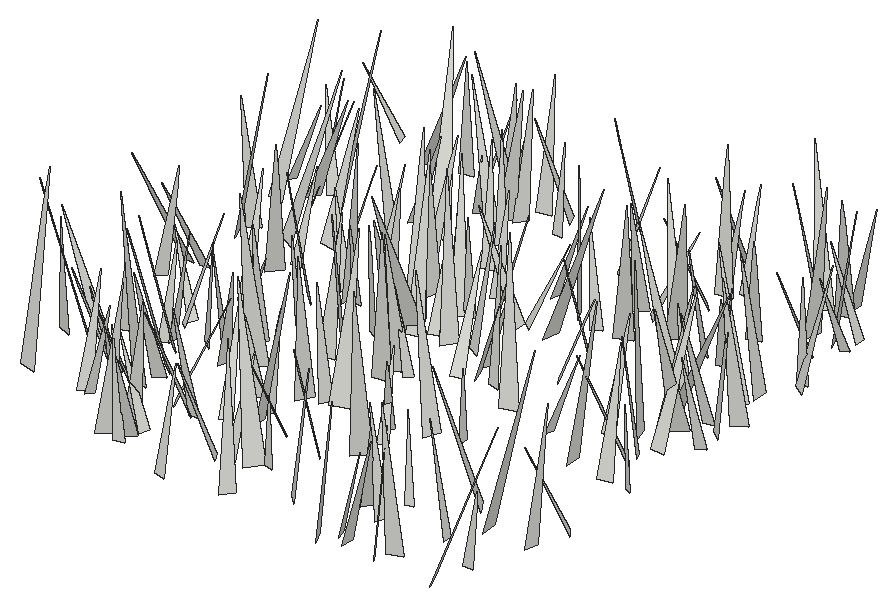
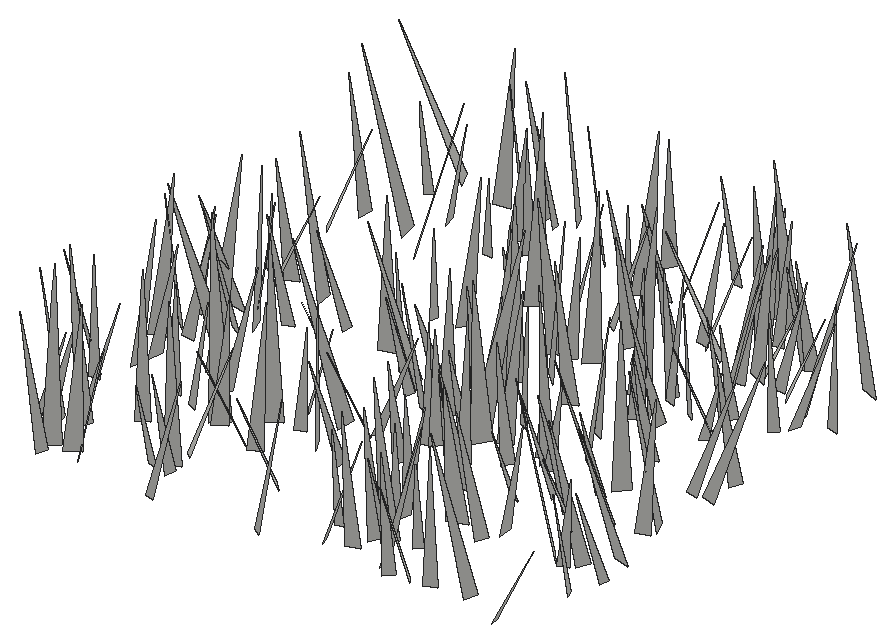
# SketchUp Ruby script. Lengths in inches.
U = 1.inch
M = Sketchup.active_model
def pt(a) = Geom::Point3d.new(a.map { |v| v * U })
def face(e, loops, mat)
  f = e.add_face(loops[0].map { |a| pt(a) })
  loops[1..].each { |l| e.add_face(l.map { |a| pt(a) }).erase! }
  f.material = f.back_material = mat if mat
  f
end
# faces: each face lists its corners as indices into pts; further lists are holes
def faces(e, pts, list, mat = nil) = list.each { |f| face(e, (f[0].is_a?(Array) ? f : [f]).map { |l| l.map { |i| pts[i] } }, mat) }
# xy, xz, yz: faces in a plane at the given z, y or x. An outline is a flat list of corners, or four numbers for a rectangle; further outlines are holes
def ring(l) = l.size == 4 ? [[l[0], l[1]], [l[2], l[1]], [l[2], l[3]], [l[0], l[3]]] : l.each_slice(2).to_a
def flat(e, list, mat, &to3) = list.each { |f| face(e, (f[0].is_a?(Array) ? f : [f]).map { |l| ring(l).map { |u, v| to3.(u, v) } }, mat) }
def xy(e, z, list, mat = nil) = flat(e, list, mat) { |x, y| [x, y, z] }
def xz(e, y, list, mat = nil) = flat(e, list, mat) { |x, z| [x, y, z] }
def yz(e, x, list, mat = nil) = flat(e, list, mat) { |y, z| [x, y, z] }
def lines(e, pts, list) = list.each { |a, b| e.add_line(pt(pts[a]), pt(pts[b])) }
# prism: a flat outline (further loops are holes) pulled along v
def prism(e, loops, v, mat = nil)
  f = face(e, loops, mat); d = Geom::Vector3d.new(v.map { |x| x * U })
  f.pushpull(f.normal.samedirection?(d) ? d.length : -d.length)
end
def box(e, o, s, mat = nil) = prism(e, [[o, [o[0] + s[0], o[1], o[2]], [o[0] + s[0], o[1] + s[1], o[2]], [o[0], o[1] + s[1], o[2]]]], [0, 0, s[2]], mat)
def at(x, y, z, deg = 0) = Geom::Transformation.translation(pt([x, y, z])) * Geom::Transformation.rotation(ORIGIN, Z_AXIS, deg.degrees)
def axes(o, x, y, z) = Geom::Transformation.new([*x, 0, *y, 0, *z, 0, *pt(o).to_a, 1])
def part(name) = M.definitions.add(name)
# library, detail: a bought-in or finely detailed component or shape, given as its bounding box
def library(name, o, s) = part(name).tap { |d| box(d.entities, o, s) }
def detail(e, o, s) = box(e.add_group.entities, o, s)
def put(e, d, t, mat = nil) = e.add_instance(d, t).tap { |i| i.material = mat if mat }
def group(e, t, mat = nil) = e.add_group.tap { |g| g.transformation = t; g.material = mat if mat }.entities
root = M.entities
c1 = part("fur_instance\#9")
p = [[0.8125,0,1.79],[0.67,-0.02,1.48],[0,-0.11,0],[0,0.11,0]]
faces(c1.entities,p,[[0,1,2,3]])
put(root,c1,axes([499.34,279.74,-21.66],[-1.38983,-5.84462,0.0201],[-5.82782,1.38425,-0.46046],[-0.44334,0.12603,5.98992]))
put(root,c1,axes([498.6,291.3,-21.66],[1.7832,7.11152,0.69499],[7.11724,-1.83129,0.47737],[-0.63379,-0.55606,7.31612]))
put(root,c1,axes([497.63,294.57,-21.66],[3.74369,-0.67268,0.40161],[-0.71907,-3.7286,0.45768],[-0.31101,0.52348,3.776]))
put(root,c1,axes([498.79,265.3,-21.66],[-1.48378,-4.80354,1.85374],[-5.06695,1.70492,0.36217],[0.91449,1.65264,5.01442]))
put(root,c1,axes([500.375,304.53,-21.66],[-3.53813,-0.73541,0.01575],[-0.72603,3.50386,0.50526],[0.11809,-0.49152,3.57826]))
put(root,c1,axes([498.56,297.67,-21.66],[3.70099,1.78589,1.07617],[1.91017,-3.78303,-0.29128],[-0.83593,-0.7377,4.09901]))
put(root,c1,axes([501.26,266.79,-21.66],[-5.40823,0.65228,0.52882],[0.69912,5.40686,0.48075],[0.46513,-0.5426,5.42617]))
put(root,c1,axes([500.03,286.84,-21.66],[1.93856,-5.12728,2.24723],[-5.46022,-2.25638,-0.43794],[-1.23493,1.9279,5.46399]))
put(root,c1,axes([499.18,276.6,-21.66],[4.20018,-2.603,1.54886],[-2.85846,-4.28223,0.55487],[-1.0019,1.30501,4.91012]))
put(root,c1,axes([500.125,259.14,-21.66],[2.12447,7.8086,2.15105],[8.03257,-2.31646,0.47574],[-1.03873,-1.94278,8.07844]))
put(root,c1,axes([500.91,279.75,-21.66],[-0.25255,-4.7231,0.0991],[-4.68784,0.23828,-0.59045],[-0.58449,0.12972,4.69284]))
put(root,c1,axes([499.63,285.33,-21.66],[6.18065,2.99725,1.89028],[2.99834,-6.44896,0.42186],[-1.88855,-0.42956,6.85609]))
put(root,c1,axes([502.44,264.21,-21.66],[-5.20648,-5.71637,1.32602],[-5.85189,5.18966,-0.6046],[0.43665,1.3904,7.70836]))
put(root,c1,axes([501.63,294.57,-21.66],[-2.18486,3.79279,1.02862],[3.92891,2.13324,0.47945],[0.08359,-1.13179,4.35074]))
put(root,c1,axes([501.34,292.31,-21.66],[4.04394,2.43918,0.42992],[2.39305,-4.06014,0.52577],[-0.63852,0.23141,4.69325]))
put(root,c1,axes([500.51,293.5,-21.66],[5.28357,-2.5058,0.04843],[-2.504,-5.27298,0.35108],[0.10676,0.33794,5.83712]))
put(root,c1,axes([502.1875,268.22,-21.66],[2.0816,-3.74764,1.04429],[-3.88491,-2.06538,0.3318],[-0.20701,1.076,4.27408]))
put(root,c1,axes([504.64,263.61,-21.66],[-3.58425,-2.16039,0.18109],[-2.16614,3.55434,-0.47063],[-0.08907,0.49634,4.15845]))
put(root,c1,axes([505.53,272.56,-21.66],[-3.05082,2.35934,0.28628],[2.37608,3.01778,0.45074],[-0.05159,-0.53147,3.83025]))
put(root,c1,axes([502.97,293.86,-21.66],[5.7382,5.20942,1.87337],[5.41352,-5.84467,-0.3291],[-1.15821,-1.50876,7.74318]))
put(root,c1,axes([503.29,286.72,-21.66],[3.5873,6.66463,1.07182],[6.75002,-3.55215,-0.50434],[-0.05834,-1.18311,7.55193]))
put(root,c1,axes([505.76,263.01,-21.66],[0.4513,-4.46287,0.47479],[-4.46772,-0.49211,-0.3789],[-0.42669,0.43236,4.4696]))
put(root,c1,axes([507.15,268.3125,-21.66],[2.82941,3.82153,3.56935],[4.50896,-3.83832,0.53527],[-2.64833,-2.45217,4.72474]))
put(root,c1,axes([505.79,258.96,-21.66],[-2.49427,4.27012,1.59064],[4.35584,2.76683,-0.59729],[1.33819,-1.04698,4.90903]))
put(root,c1,axes([505.79,268.68,-21.66],[2.7326,-2.75522,2.01665],[-3.2693,-2.85632,0.52755],[-0.98478,1.83723,3.84448]))
put(root,c1,axes([505.4,271.625,-21.66],[2.99735,3.72962,0.28981],[3.68324,-3.00724,0.60693],[-0.65404,0.15682,4.74613]))
put(root,c1,axes([506.6875,277.54,-21.66],[-1.85743,4.94831,0.92273],[4.99711,1.93095,-0.29602],[0.60509,-0.75691,5.27714]))
put(root,c1,axes([506.23,284.25,-21.66],[-0.0874,4.08723,0.80677],[4.1529,0.14964,-0.30818],[0.33125,-0.79758,4.07653]))
put(root,c1,axes([506.19,269.28,-21.66],[4.45017,0.43948,1.54669],[0.28501,-4.6951,0.51402],[-1.58245,0.39027,4.44218]))
put(root,c1,axes([505.49,282.6,-21.66],[5.14782,-4.26055,1.16689],[-4.27581,-5.25589,-0.32723],[-1.10966,0.4872,6.67423]))
put(root,c1,axes([508.16,261.84,-21.66],[-3.2308,-2.41105,0.08917],[-2.40238,3.20101,-0.49122],[-0.22293,0.4467,4.00124]))
put(root,c1,axes([504.15,302.67,-21.66],[6.51578,-0.90085,0.09034],[-0.89347,-6.50413,-0.41604],[-0.1463,-0.39981,6.56459]))
put(root,c1,axes([506.24,288.07,-21.66],[-0.03084,5.75903,1.17934],[5.85206,0.14189,-0.53988],[0.55736,-1.17118,5.73375]))
put(root,c1,axes([508.36,293.22,-21.66],[-5.56537,0.35389,1.01892],[0.25962,5.63719,-0.53984],[1.04691,0.48332,5.55042]))
put(root,c1,axes([506.39,258.94,-21.66],[3.89931,-1.45547,0.98195],[-1.58431,-3.9476,0.44006],[-0.75669,0.76505,4.13877]))
put(root,c1,axes([508.73,265.49,-21.66],[-4.07714,-4.72232,1.18622],[-4.85623,4.056,-0.54439],[0.3528,1.25658,6.21506]))
put(root,c1,axes([508.3125,262.53,-21.66],[-2.90002,-7.26429,3.03178],[-7.85451,2.88308,-0.60516],[0.51793,3.0479,7.79832]))
put(root,c1,axes([507.6,303.32,-21.66],[1.5026,-5.2869,1.47769],[-5.48951,-1.44343,0.41772],[0.01326,1.53554,5.48039]))
put(root,c1,axes([508.99,264.18,-21.66],[1.67149,-5.33301,0.8085],[-5.34441,-1.75188,-0.5067],[-0.72935,0.6152,5.5658]))
put(root,c1,axes([508.61,270.39,-21.66],[2.85129,3.39796,1.84964],[3.79237,-2.9092,-0.50161],[-0.76499,-1.75715,4.40731]))
put(root,c1,axes([510.35,280.75,-21.66],[-3.95359,-4.39819,1.62013],[-4.4402,4.19331,0.54823],[1.50116,0.81969,5.8885]))
put(root,c1,axes([509.02,286.45,-21.66],[4.30125,1.72732,0.68489],[1.69718,-4.35514,0.32517],[-0.75649,0.05042,4.6237]))
put(root,c1,axes([509.4,303.49,-21.66],[3.16954,2.48643,0.53995],[2.54162,-3.13416,-0.48689],[-0.1185,-0.71733,3.99891]))
put(root,c1,axes([510.1,257.78,-21.66],[0.02895,-4.95019,0.58964],[-4.94989,0.0415,0.59139],[0.59214,0.58889,4.91483]))
put(root,c1,axes([512.21,294.27,-21.66],[-3.14428,7.71271,0.49149],[7.72648,3.12546,0.38342],[-0.17032,-0.59964,8.32018]))
put(root,c1,axes([509.08,295.21,-21.66],[4.36325,-2.68491,0.18726],[-2.69098,-4.34538,0.39756],[0.04948,0.43666,5.1077]))
put(root,c1,axes([511.69,283.57,-21.66],[-3.05036,2.77962,1.08054],[2.93347,3.07501,0.37088],[0.53722,-1.00823,4.11016]))
put(root,c1,axes([511.12,288.67,-21.66],[1.03899,3.82207,0.22987],[3.79032,-1.06041,0.49963],[-0.54276,-0.08876,3.92914]))
put(root,c1,axes([509.55,272.8125,-21.66],[4.16125,-1.09144,0.28201],[-1.11074,-4.15389,0.31328],[-0.19241,0.37504,4.29058]))
put(root,c1,axes([512.47,302.75,-21.66],[-6.25427,-0.78477,1.30734],[-0.71032,6.38344,0.43371],[1.34924,-0.27711,6.28838]))
put(root,c1,axes([511.19,269.66,-21.66],[-1.65824,-4.82946,1.36253],[-4.95542,1.80194,0.35604],[0.78993,1.16588,5.09379]))
put(root,c1,axes([510.92,272.39,-21.66],[4.15437,2.45212,1.76514],[2.75663,-4.30471,-0.50784],[-1.23677,-1.35794,4.79727]))
put(root,c1,axes([512.28,277.05,-21.66],[0.90627,3.33198,1.59944],[3.57947,-1.20149,0.47479],[-0.9207,-1.39138,3.42023]))
put(root,c1,axes([511.11,303.9375,-21.66],[3.01124,-3.84874,1.35887],[-4.04465,-3.04041,0.35153],[-0.54781,1.29229,4.87409]))
put(root,c1,axes([513.33,256.85,-21.66],[-4.0044,1.49429,0.5536],[1.5481,4.00291,0.3933],[0.37782,-0.56428,4.25599]))
put(root,c1,axes([511.1,254.85,-21.66],[5.02607,-4.57327,2.19343],[-4.92834,-5.13329,0.59007],[-1.19892,1.92923,6.76964]))
put(root,c1,axes([511.59,273.23,-21.66],[4.45698,-3.93649,1.376],[-3.92382,-4.64074,-0.56675],[-1.41173,0.47074,5.91941]))
put(root,c1,axes([512.8125,254.48,-21.66],[-0.34045,4.62028,2.07312],[5.05885,0.21591,0.34957],[-0.23002,-2.08976,4.6196]))
put(root,c1,axes([511.52,268.94,-21.66],[4.68677,-2.0034,0.66372],[-1.95488,-4.73014,-0.47351],[-0.79535,-0.17932,5.07496]))
put(root,c1,axes([511.71,257.5,-21.66],[3.13383,-5.16211,1.39491],[-5.34355,-3.08346,0.59403],[-0.19921,1.50298,6.00961]))
put(root,c1,axes([512,299.24,-21.66],[1.97582,-3.11414,0.08334],[-3.10691,-1.9626,0.3224],[0.22782,0.24287,3.67393]))
put(root,c1,axes([514.36,261.22,-21.66],[-3.87512,-3.17972,0.32504],[-3.163,3.88842,0.32938],[0.4601,-0.04943,5.00187]))
put(root,c1,axes([512.65,282.7,-21.66],[7.01983,-0.71592,2.31882],[-0.6287,-7.39114,-0.37866],[-2.34397,-0.1616,7.04608]))
put(root,c1,axes([513,255.68,-21.66],[2.62732,-3.98087,0.28129],[-3.95197,-2.64215,-0.47983],[-0.55532,-0.03119,4.74551]))
put(root,c1,axes([513.67,270.21,-21.66],[3.74176,-6.61768,2.63887],[-6.89022,-4.11933,-0.5604],[-1.81167,1.99888,7.58159]))
put(root,c1,axes([515.92,296.26,-21.66],[-6.2227,2.39174,0.32304],[2.36421,6.22042,-0.51348],[0.48507,0.36431,6.64671]))
put(root,c1,axes([513.51,282.51,-21.66],[0.0585,-4.06465,0.78718],[-4.11626,0.02739,0.44734],[0.44434,0.78888,4.04038]))
put(root,c1,axes([513.74,300.85,-21.66],[3.88682,0.49651,1.01606],[0.42112,-4.01087,0.34905],[-1.04955,0.22945,3.90283]))
put(root,c1,axes([514.86,261.0625,-21.66],[-0.19276,-5.01478,1.27598],[-5.16585,0.1124,-0.33865],[-0.30027,1.28555,5.00705]))
put(root,c1,axes([512.35,261.91,-21.66],[4.96423,2.67259,0.04648],[2.6631,-4.93667,-0.5706],[0.22978,-0.52435,5.60898]))
put(root,c1,axes([514.63,289.91,-21.66],[0.44242,5.64748,1.29703],[5.78226,-0.34572,-0.46699],[0.37666,-1.32609,5.6455]))
put(root,c1,axes([514.82,284.81,-21.66],[3.66382,-3.28739,1.57998],[-3.52995,-3.75957,0.36325],[-0.918,1.33625,4.90903]))
put(root,c1,axes([514.3125,299.79,-21.66],[4.31409,-4.88001,1.43702],[-5.06352,-4.30068,0.59646],[-0.49016,1.47666,6.48614]))
put(root,c1,axes([515.33,300.26,-21.66],[-4.36102,2.95909,2.58691],[3.11538,4.95832,-0.41976],[2.39639,-1.06094,5.25343]))
put(root,c1,axes([516.44,296.43,-21.66],[-4.17339,1.81444,1.20525],[1.74242,4.34394,-0.50613],[1.30721,0.0026,4.52253]))
put(root,c1,axes([515.98,302.31,-21.66],[-1.18817,5.57554,2.26119],[5.96275,1.39894,-0.31626],[0.80332,-2.13721,5.69196]))
put(root,c1,axes([517.04,262.19,-21.66],[-2.44616,4.11048,0.29857],[4.09909,2.46258,-0.31948],[0.42742,-0.0923,4.7726]))
put(root,c1,axes([516.91,266.66,-21.66],[1.11597,-3.30458,1.27259],[-3.40234,-1.37051,-0.57526],[-0.98175,0.99326,3.44016]))
put(root,c1,axes([518.3,302.8,-21.66],[-4.34148,-1.68145,0.56308],[-1.64517,4.37512,0.38015],[0.66161,-0.1544,4.64018]))
put(root,c1,axes([517.9375,292.89,-21.66],[-0.91047,5.0165,1.03079],[5.11456,0.83694,0.44447],[-0.2628,-1.09133,5.07905]))
put(root,c1,axes([516.94,274.58,-21.66],[-1.46748,5.77462,2.34569],[6.13429,1.76496,-0.50731],[1.10405,-2.13089,5.93652]))
put(root,c1,axes([517.21,287.24,-21.66],[5.69628,-2.00129,2.37758],[-1.98509,-6.1627,-0.4314],[-2.39112,0.34864,6.02217]))
put(root,c1,axes([517.49,279.49,-21.66],[-2.05605,-4.2865,1.82271],[-4.5186,2.31917,0.35698],[1.13077,1.47345,4.74068]))
put(root,c1,axes([516.99,282.44,-21.66],[3.45501,-4.88886,0.26504],[-4.85303,-3.46254,-0.60598],[-0.64754,-0.13474,5.95575]))
put(root,c1,axes([518.46,283.43,-21.66],[-5.59489,5.13542,2.2708],[5.22691,5.9344,-0.54239],[2.05147,-1.11455,7.57503]))
put(root,c1,axes([518.95,287.1,-21.66],[-3.597,-0.64897,1.74683],[-0.97146,3.89365,-0.55385],[1.59023,0.91068,3.61287]))
put(root,c1,axes([518.55,252.1875,-21.66],[0.78552,4.64999,1.51438],[4.88897,-0.70993,-0.35606],[0.11721,-1.55126,4.70241]))
put(root,c1,axes([520.07,257.15,-21.66],[-3.91317,-2.34388,0.53173],[-2.28614,3.94348,0.55853],[0.74167,-0.21123,4.52711]))
put(root,c1,axes([518.89,300.26,-21.66],[0.06663,3.86387,1.64805],[4.18879,0.06273,-0.31643],[0.31563,-1.6482,3.85147]))
put(root,c1,axes([520.09,281.39,-21.66],[-1.2461,7.24945,1.28302],[7.36015,1.19663,0.38699],[-0.1701,-1.32928,7.34558]))
put(root,c1,axes([518.94,265.03,-21.66],[-3.54773,2.23846,2.32232],[2.39169,4.14191,-0.33862],[2.16418,-0.90784,4.1812]))
put(root,c1,axes([520.79,285.88,-21.66],[-4.49131,4.50007,0.95246],[4.50728,4.57122,-0.34355],[0.91773,-0.42777,6.34858]))
put(root,c1,axes([520.58,272.4,-21.66],[3.92843,5.06138,3.38638],[5.5366,-4.64662,0.52215],[-2.53598,-2.30413,6.38572]))
put(root,c1,axes([519.85,281.875,-21.66],[2.00321,-7.73932,0.37509],[-7.71802,-2.02729,-0.61059],[-0.68548,0.20889,7.97102]))
put(root,c1,axes([519.69,268.52,-21.66],[-4.92901,3.2655,3.81824],[4.17297,5.6397,0.56365],[2.798,-2.65855,5.88565]))
put(root,c1,axes([519.32,263.49,-21.66],[6.35559,1.23086,1.81432],[1.1106,-6.60444,0.5901],[-1.89033,0.25813,6.44673]))
put(root,c1,axes([521.14,282.32,-21.66],[-1.57636,3.66287,0.67143],[3.67727,1.64614,-0.34684],[0.58749,-0.47537,3.97256]))
put(root,c1,axes([521.26,269.1,-21.66],[-4.23654,2.45749,2.21286],[2.8358,4.54981,0.37637],[1.70124,-1.46429,4.88322]))
put(root,c1,axes([521.87,263.35,-21.66],[-2.1706,-3.79382,0.07549],[-3.76138,2.16267,0.53397],[0.50075,-0.20018,4.33814]))
put(root,c1,axes([521.38,289.77,-21.66],[2.89571,-2.97183,2.13904],[-3.49598,-3.05481,0.48854],[-1.08874,1.90494,4.12046]))
put(root,c1,axes([521.2,257.49,-21.66],[0.22863,4.55848,1.01522],[4.65358,-0.13679,-0.43379],[0.39321,-1.03161,4.54355]))
put(root,c1,axes([521.46,286.34,-21.66],[0.51611,-4.80053,1.29544],[-4.96034,-0.40702,0.46794],[0.34389,1.33374,4.80546]))
put(root,c1,axes([523.23,257.95,-21.66],[-5.88987,4.84378,2.23578],[5.14185,6.04195,0.45575],[1.42207,-1.78441,7.61217]))
put(root,c1,axes([523.01,281.93,-21.66],[-6.12251,3.37612,2.03098],[3.42132,6.417,-0.35327],[1.95387,-0.65732,6.98272]))
put(root,c1,axes([522.54,269.16,-21.66],[-2.30774,6.81626,2.09214],[7.04491,2.51871,-0.43516],[1.09893,-1.8327,7.18315]))
put(root,c1,axes([522.82,276.3,-21.66],[2.11565,-6.08651,1.80009],[-6.2822,-2.27872,-0.32139],[-0.90548,1.58863,6.43571]))
put(root,c1,axes([523.21,304.9,-21.66],[-3.17607,-4.40082,1.193],[-4.40846,3.33508,0.56622],[1.16445,0.62283,5.3976]))
put(root,c1,axes([523.72,276.03,-21.66],[1.42768,-3.34431,1.65268],[-3.54003,-1.77266,-0.52903],[-1.17641,1.27565,3.59761]))
put(root,c1,axes([522.42,274.41,-21.66],[2.16747,-6.96935,1.82134],[-7.20329,-2.08612,0.58967],[0.04123,1.91397,7.27476]))
put(root,c1,axes([525.48,287.36,-21.66],[-5.10669,0.68056,0.36828],[0.71376,5.09217,0.48729],[0.29888,-0.53268,5.12875]))
put(root,c1,axes([524.3,253.25,-21.66],[-5.32179,3.05618,1.70346],[3.04909,5.5718,-0.47069],[1.71611,-0.42222,6.11884]))
put(root,c1,axes([524.18,258.44,-21.66],[-0.14412,-3.47359,1.04669],[-3.58722,0.2928,0.47779],[0.54152,1.01518,3.44359]))
put(root,c1,axes([526.11,262.19,-21.66],[-3.38614,-3.10021,1.02366],[-3.22386,3.40798,-0.34286],[0.51569,0.94841,4.57818]))
put(root,c1,axes([525.09,282.25,-21.66],[2.3418,4.95634,1.60959],[5.19702,-2.35112,-0.32146],[-0.38351,-1.59595,5.4723]))
put(root,c1,axes([524.69,292.75,-21.66],[4.46137,-0.22154,0.62784],[-0.29219,-4.4737,0.49769],[-0.59824,0.53291,4.43905]))
put(root,c1,axes([526.66,278.35,-21.66],[-2.17484,4.53028,0.06229],[4.50087,2.16823,-0.54601],[0.51907,0.1805,4.99552]))
put(root,c1,axes([526.32,298.43,-21.66],[3.1839,3.43631,0.24845],[3.39454,-3.18669,0.57383],[-0.5891,0.20968,4.64932]))
put(root,c1,axes([525.89,287.86,-21.66],[2.47782,3.1575,0.0552],[3.13992,-2.45577,-0.47176],[0.33732,-0.3344,3.98583]))
put(root,c1,axes([527.96,291.64,-21.66],[5.01686,3.02729,2.73746],[3.17963,-5.61852,0.38618],[-2.55892,-1.04628,5.84673]))
put(root,c1,axes([528.7,266.75,-21.66],[-2.71022,2.78687,0.60598],[2.7235,2.77712,-0.59105],[0.8464,-0.01233,3.84222]))
put(root,c1,axes([527.74,268.65,-21.66],[3.24769,-2.54753,0.32293],[-2.51539,-3.26077,-0.4265],[-0.51676,-0.13836,4.10555]))
put(root,c1,axes([527.39,281.01,-21.66],[3.65064,-1.60023,0.53489],[-1.66152,-3.63138,0.47591],[-0.29361,0.65299,3.95745]))
put(root,c1,axes([528.51,264.31,-21.66],[5.1556,-5.75467,2.21602],[-5.90961,-5.43588,-0.36737],[-1.76168,1.39363,7.71761]))
put(root,c1,axes([528.6875,255.78,-21.66],[4.00395,3.96639,1.91354],[4.25291,-4.1539,-0.28869],[-1.14309,-1.56151,5.62855]))
put(root,c1,axes([527.76,279.45,-21.66],[6.78168,2.91502,1.19431],[2.8839,-6.88568,0.43057],[-1.26762,-0.07012,7.36906]))
put(root,c1,axes([529.69,278.96,-21.66],[1.56528,5.39191,1.82425],[5.61252,-1.77733,0.43748],[-0.9488,-1.61836,5.59744]))
put(root,c1,axes([530.79,270.1,-21.66],[-6.02179,2.8816,2.13168],[3.11245,6.27078,0.31555],[1.77772,-1.21792,6.66828]))
put(root,c1,axes([530.41,290.62,-21.66],[1.59272,-3.9303,2.28796],[-4.37909,-1.9795,-0.352],[-1.22702,1.96293,4.22612]))
put(root,c1,axes([528.25,287.73,-21.66],[7.76844,-0.71206,0.72464],[-0.74639,-7.79129,0.34557],[-0.68922,0.41169,7.79335]))
put(root,c1,axes([531.84,287.8,-21.66],[-3.00946,-2.45302,0.73779],[-2.54129,3.00205,-0.38468],[0.32167,0.76736,3.86344]))
put(root,c1,axes([531.17,295.16,-21.66],[3.50702,-4.68842,0.88051],[-4.69288,-3.58696,-0.4079],[-0.85643,0.45629,5.84073]))
put(root,c1,axes([532.91,276.88,-21.66],[-2.11891,6.73628,2.3501],[7.12334,2.13432,0.30482],[0.39806,-2.33612,7.05509]))
put(root,c1,axes([532.98,305.82,-21.66],[-1.82356,-4.42835,0.39133],[-4.41286,1.85435,0.42054],[0.53859,0.19978,4.77062]))
put(root,c1,axes([533.3,270.75,-21.66],[3.51099,-0.42801,1.09439],[-0.295,-3.65871,-0.48452],[-1.13748,-0.37227,3.50364]))
put(root,c1,axes([534.71,298.82,-21.66],[-3.28468,-3.33783,0.1825],[-3.30088,3.27904,0.56182],[0.52783,-0.26523,4.64915]))
put(root,c1,axes([533.04,282.66,-21.66],[3.15167,2.15202,0.19961],[2.1362,-3.1554,0.29004],[-0.32814,0.12762,3.80527]))
put(root,c1,axes([532.47,294.83,-21.66],[3.00056,3.161,0.00616],[3.13284,-2.97269,-0.58633],[0.42105,-0.40809,4.31874]))
put(root,c1,axes([532.87,290.84,-21.66],[3.4393,-6.56896,1.063],[-6.65437,-3.3911,0.57422],[0.02233,1.20797,7.39258]))
put(root,c1,axes([533.98,301.94,-21.66],[3.92282,-1.4058,1.44453],[-1.66907,-4.03753,0.60333],[-1.1301,1.0833,4.1232]))
put(root,c1,axes([535.75,293.73,-21.66],[2.97491,-4.25566,3.74848],[-5.0806,-3.88069,-0.37363],[-2.51977,2.80026,5.17891]))
put(root,c1,axes([533.94,252.29,-21.66],[5.56182,2.46032,2.03104],[2.73268,-5.78042,-0.48104],[-1.64644,-1.28288,6.06264]))
put(root,c1,axes([534.66,300.84,-21.66],[-1.49682,6.02983,3.22428],[6.74332,1.8484,-0.32627],[1.1325,-3.03643,6.20426]))
put(root,c1,axes([533.81,258.48,-21.66],[3.85722,-2.97975,0.1804],[-2.96484,-3.85827,-0.33622],[-0.3481,-0.15623,4.86251]))
put(root,c1,axes([535.79,301.85,-21.66],[0.78964,4.34465,0.57519],[4.335,-0.86018,0.54605],[-0.64386,-0.46311,4.38193]))
put(root,c1,axes([536.03,257.47,-21.66],[-4.24357,2.27798,1.78244],[2.54082,4.44811,0.36434],[1.38223,-1.18292,4.80254]))
put(root,c1,axes([536.3,260.5,-21.66],[-0.50007,3.75556,1.02909],[3.87876,0.38868,0.46638],[-0.34425,-1.07612,3.75989]))
put(root,c1,axes([534.99,253.83,-21.66],[3.94564,1.0984,0.79467],[1.2,-3.96752,-0.47419],[-0.63087,-0.67703,4.06813]))
put(root,c1,axes([538.45,289.58,-21.66],[-6.00997,1.04438,1.22572],[1.13938,6.10462,0.38513],[1.13796,-0.59647,6.08787]))
put(root,c1,axes([536.19,253.07,-21.66],[5.46664,-0.56538,0.68203],[-0.51758,-5.49848,-0.40957],[-0.71898,-0.34055,5.48051]))
put(root,c1,axes([536,293.37,-21.66],[5.23004,-6.31048,0.45418],[-6.32662,-5.22094,0.31214],[-0.04891,0.54893,8.19012]))
put(root,c1,axes([539.24,292.85,-21.66],[1.51862,3.68557,2.40948],[4.21899,-1.94756,0.31991],[-1.2606,-2.07817,3.97332]))
put(root,c1,axes([537.43,276.08,-21.66],[4.04534,-0.8517,0.30361],[-0.87788,-4.03293,0.38361],[-0.21657,0.43867,4.11619]))
put(root,c1,axes([539.22,252.55,-21.66],[-4.16278,-2.64249,2.71758],[-3.23685,4.57857,-0.50613],[1.97251,1.93665,4.90462]))
put(root,c1,axes([540.73,263.81,-21.66],[-5.52316,-3.7636,0.965],[-3.71814,5.60658,0.58551],[1.12752,0.05244,6.65787]))
put(root,c1,axes([540.9375,304.43,-21.66],[-4.28874,-2.62611,1.19653],[-2.76089,4.3576,-0.33198],[0.84,0.91449,5.01792]))
put(root,c1,axes([540.22,253.82,-21.66],[1.19646,-6.35488,2.45253],[-6.76034,-1.41301,-0.36331],[-0.83491,2.33448,6.45631]))
put(root,c1,axes([541.83,258.18,-21.66],[-4.7779,-0.84592,1.0787],[-0.97294,4.84801,-0.50762],[0.9657,0.69908,4.82558]))
put(root,c1,axes([541.32,287.83,-21.66],[1.53479,-3.08573,1.52348],[-3.30012,-1.79268,-0.30636],[-0.97569,1.2095,3.43271]))
put(root,c1,axes([541.95,303.92,-21.66],[-4.3858,5.26104,2.02142],[5.54364,4.48874,0.34523],[1.01623,-1.78118,6.84066]))
put(root,c1,axes([541.33,278.45,-21.66],[-0.63443,5.02312,1.44392],[5.17666,0.80438,-0.52377],[0.72032,-1.3566,5.03586]))
put(root,c1,axes([540.72,296.92,-21.66],[2.46673,-5.38252,0.46134],[-5.39282,-2.42347,0.55987],[0.31917,0.65147,5.89431]))
put(root,c1,axes([541.33,292.26,-21.66],[1.84889,-3.8875,0.07331],[-3.87281,-1.83403,0.41727],[0.34554,0.24513,4.2845]))
put(root,c1,axes([541.73,273.59,-21.66],[7.00703,0.38351,2.14023],[0.30488,-7.32356,0.31416],[-2.15283,0.21111,7.01048]))
put(root,c1,axes([543.16,280.04,-21.66],[-6.66859,-2.01923,2.71074],[-2.32845,7.09045,-0.44648],[2.45024,1.24248,6.95328]))
put(root,c1,axes([545.35,275.9,-21.66],[-3.79986,-3.34827,0.10157],[-3.34083,3.7767,-0.4853],[-0.24505,0.43103,5.04126]))
put(root,c1,axes([545.08,277.36,-21.66],[-4.18009,-2.38384,1.39005],[-2.61185,4.23208,-0.59649],[0.8906,1.22265,4.77494]))
put(root,c1,axes([543.9,281.54,-21.66],[2.83544,5.2975,1.05869],[5.3487,-2.92083,0.29014],[-0.75876,-0.79328,6.00159]))
put(root,c1,axes([546.26,288.4375,-21.66],[-6.22467,1.67352,0.58559],[1.62437,6.23957,-0.56507],[0.71064,0.39649,6.42089]))
put(root,c1,axes([543.33,261.41,-21.66],[8.05424,1.38868,1.7961],[1.29513,-8.24767,0.56905],[-1.86468,0.26973,8.15325]))
put(root,c1,axes([545.46,297.88,-21.66],[-2.21382,-3.77344,0.32599],[-3.76288,2.23425,0.30817],[0.43109,0.1241,4.36404]))
put(root,c1,axes([543.75,300.23,-21.66],[6.97924,-1.80721,1.76653],[-1.77915,-7.19853,-0.33521],[-1.79479,0.10824,7.20163]))
put(root,c1,axes([543.86,304.13,-21.66],[3.44417,-6.15496,0.43731],[-6.17002,-3.42915,0.33004],[0.07525,0.54268,7.04535]))
put(root,c1,axes([543.71,305.48,-21.66],[5.53978,-0.90724,0.62547],[-0.85463,-5.56113,-0.49688],[-0.69563,-0.39269,5.59154]))
put(root,c1,axes([545.49,272.83,-21.66],[-2.00411,5.21831,1.67163],[5.38658,2.20263,-0.41796],[1.00489,-1.39973,5.57427]))
put(root,c1,axes([546.15,284.66,-21.66],[0.08099,-5.17118,1.20761],[-5.27072,-0.22549,-0.61212],[-0.64729,1.18913,5.13546]))
put(root,c1,axes([545.11,282.4,-21.66],[3.26606,-6.16963,0.62937],[-6.14796,-3.31446,-0.58694],[-0.81426,0.27855,6.95607]))
put(root,c1,axes([543.04,284.46,-21.66],[6.75875,-1.16964,0.00047],[-1.16859,-6.75255,0.29358],[0.0496,0.28936,6.85293]))
put(root,c1,axes([545.83,278.81,-21.66],[0.77683,6.56918,0.32302],[6.56801,-0.79193,0.30978],[-0.34589,-0.28401,6.60769]))
put(root,c1,axes([547.17,301.73,-21.66],[-4.29082,0.07848,0.62907],[0.12494,4.3243,0.31276],[0.62151,-0.32753,4.28013]))
put(root,c1,axes([546.57,290.34,-21.66],[5.59524,-0.57904,3.08549],[-0.36766,-6.38318,-0.53118],[-3.11775,-0.28642,5.59999]))
put(root,c1,axes([545.76,255.8,-21.66],[0.94774,-3.5048,1.15841],[-3.67796,-0.79512,0.60341],[0.31324,1.26803,3.58018]))
put(root,c1,axes([545.68,300.55,-21.66],[5.68987,2.39384,1.65752],[2.61602,-5.80047,-0.60296],[-1.2784,-1.21517,6.14342]))
put(root,c1,axes([547.16,299.96,-21.66],[0.58704,-3.79537,0.45103],[-3.78334,-0.64184,-0.47675],[-0.5428,0.36891,3.81079]))
put(root,c1,axes([545.04,252.34,-21.66],[6.72288,3.05704,0.61475],[3.02645,-6.7488,0.46346],[-0.75102,0.16938,7.37074]))
put(root,c1,axes([548.42,264.88,-21.66],[-3.47143,-2.84551,0.09651],[-2.81271,3.45107,0.57956],[0.4415,-0.38766,4.45106]))
put(root,c1,axes([547.79,272.74,-21.66],[1.56672,2.93333,1.48069],[3.11219,-1.85095,0.37383],[-1.05412,-1.105,3.30444]))
put(root,c1,axes([547.71,283.57,-21.66],[3.73887,4.62596,1.90486],[4.75099,-4.02818,0.45718],[-1.5672,-1.17533,5.9304]))
put(root,c1,axes([548.09,281.23,-21.66],[1.30026,-4.12004,1.09762],[-4.18224,-1.45572,-0.50983],[-0.82967,0.8811,4.29016]))
put(root,c1,axes([547.53,261.27,-21.66],[5.90361,-0.69248,2.28384],[-0.937,-6.27702,0.51884],[-2.19488,0.81708,5.9214]))
put(root,c1,axes([548.19,285.84,-21.66],[-2.64442,5.36733,3.49605],[6.32318,2.79183,0.49668],[1.02376,-3.3795,5.96276]))
put(root,c1,axes([547.81,293.95,-21.66],[0.13174,-4.85064,1.64659],[-5.10405,0.01535,0.4536],[0.43432,1.65178,4.83118]))
put(root,c1,axes([548.24,293,-21.66],[2.85218,4.71528,1.10181],[4.83661,-2.83604,-0.38317],[-0.23454,-1.14272,5.49745]))
